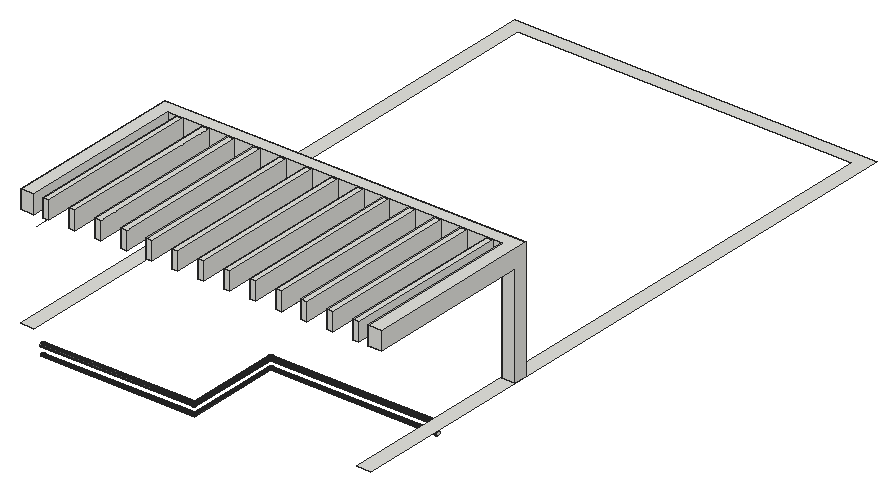
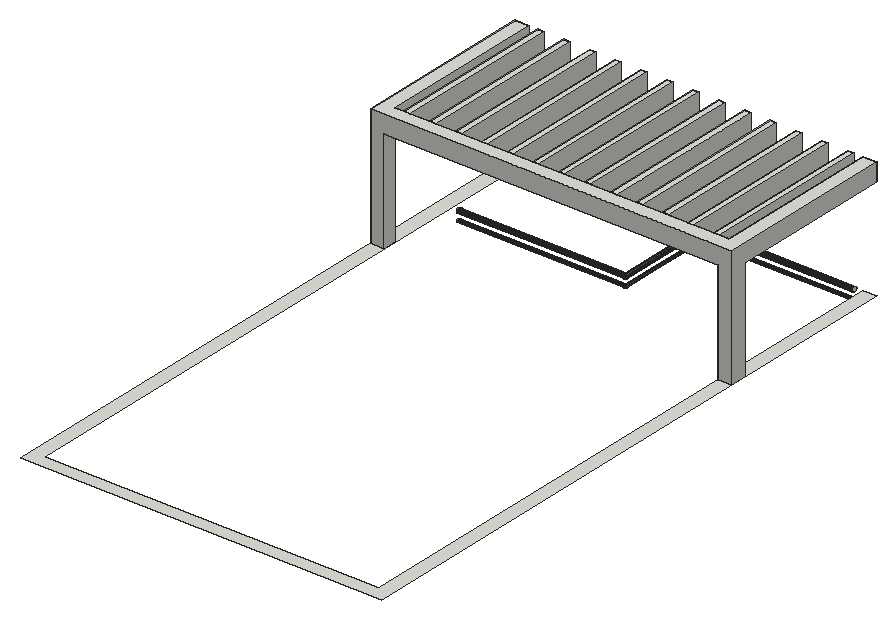
# SketchUp Ruby script. Lengths in inches.
U = 1.inch
M = Sketchup.active_model
def pt(a) = Geom::Point3d.new(a.map { |v| v * U })
def face(e, loops, mat)
  f = e.add_face(loops[0].map { |a| pt(a) })
  loops[1..].each { |l| e.add_face(l.map { |a| pt(a) }).erase! }
  f.material = f.back_material = mat if mat
  f
end
# faces: each face lists its corners as indices into pts; further lists are holes
def faces(e, pts, list, mat = nil) = list.each { |f| face(e, (f[0].is_a?(Array) ? f : [f]).map { |l| l.map { |i| pts[i] } }, mat) }
# xy, xz, yz: faces in a plane at the given z, y or x. An outline is a flat list of corners, or four numbers for a rectangle; further outlines are holes
def ring(l) = l.size == 4 ? [[l[0], l[1]], [l[2], l[1]], [l[2], l[3]], [l[0], l[3]]] : l.each_slice(2).to_a
def flat(e, list, mat, &to3) = list.each { |f| face(e, (f[0].is_a?(Array) ? f : [f]).map { |l| ring(l).map { |u, v| to3.(u, v) } }, mat) }
def xy(e, z, list, mat = nil) = flat(e, list, mat) { |x, y| [x, y, z] }
def xz(e, y, list, mat = nil) = flat(e, list, mat) { |x, z| [x, y, z] }
def yz(e, x, list, mat = nil) = flat(e, list, mat) { |y, z| [x, y, z] }
def lines(e, pts, list) = list.each { |a, b| e.add_line(pt(pts[a]), pt(pts[b])) }
# prism: a flat outline (further loops are holes) pulled along v
def prism(e, loops, v, mat = nil)
  f = face(e, loops, mat); d = Geom::Vector3d.new(v.map { |x| x * U })
  f.pushpull(f.normal.samedirection?(d) ? d.length : -d.length)
end
def box(e, o, s, mat = nil) = prism(e, [[o, [o[0] + s[0], o[1], o[2]], [o[0] + s[0], o[1] + s[1], o[2]], [o[0], o[1] + s[1], o[2]]]], [0, 0, s[2]], mat)
def at(x, y, z, deg = 0) = Geom::Transformation.translation(pt([x, y, z])) * Geom::Transformation.rotation(ORIGIN, Z_AXIS, deg.degrees)
def axes(o, x, y, z) = Geom::Transformation.new([*x, 0, *y, 0, *z, 0, *pt(o).to_a, 1])
def part(name) = M.definitions.add(name)
# library, detail: a bought-in or finely detailed component or shape, given as its bounding box
def library(name, o, s) = part(name).tap { |d| box(d.entities, o, s) }
def detail(e, o, s) = box(e.add_group.entities, o, s)
def put(e, d, t, mat = nil) = e.add_instance(d, t).tap { |i| i.material = mat if mat }
def group(e, t, mat = nil) = e.add_group.tap { |g| g.transformation = t; g.material = mat if mat }.entities
root = M.entities
M.materials.add("[Color M05]").color = [114, 114, 114]
xy(root,307.1,[[231,223.5,240,223.5,240,643.5,0,643.5,0,232.5,9,232.5,9,634.5,231,634.5],[0,341.375,9,352.5],[231,343.5,240,352.5]])
xy(root,375.1,[[0,232.5,9,341.375],[231,232.5,240,343.5],[9,343.5,231,352.5]])
xy(root,387.1,[[0,232.5,9,232.5,9,343.5,231,343.5,231,232.5,240,232.5,240,352.5,0,352.5]])
xz(root,232.5,[[0,375.1,9,387.1],[231,375.1,240,387.1]])
xz(root,341.375,[[0,307.1,9,375.1]])
xz(root,343.5,[[231,307.1,240,375.1],[9,375.1,15,387.1],[19,375.1,231,387.1]])
xz(root,352.5,[[0,307.1,0,387.1,240,387.1,240,307.1,231,307.1,231,375.1,9,375.1,9,307.1]])
yz(root,0,[[341.375,307.1,341.375,375.1,232.5,375.1,232.5,387.1,352.5,387.1,352.5,307.1]])
yz(root,9,[[341.375,307.1,352.5,307.1,352.5,375.1,343.5,375.1,343.5,387.1,232.5,387.1,232.5,375.1,341.375,375.1]])
yz(root,18,[[228,295.92,227.74,295.95,227.5,296.05,227.29,296.21,227.13,296.42,227.03,296.66,227,296.92,227.03,297.18,227.13,297.42,227.29,297.625,227.5,297.78,227.74,297.88,228,297.92,228.26,297.88,228.5,297.78,228.71,297.625,228.87,297.42,228.97,297.18,229,296.92,228.97,296.66,228.87,296.42,228.71,296.21,228.5,296.05,228.26,295.95],[228,301.42,227.61,301.47,227.25,301.62,226.9375,301.86,226.7,302.17,226.55,302.53,226.5,302.92,226.55,303.31,226.7,303.67,226.9375,303.98,227.25,304.22,227.61,304.37,228,304.42,228.39,304.37,228.75,304.22,229.0625,303.98,229.3,303.67,229.45,303.31,229.5,302.92,229.45,302.53,229.3,302.17,229.0625,301.86,228.75,301.62,228.39,301.47]])
yz(root,231,[[291,295.92,291.26,295.95,291.5,296.05,291.71,296.21,291.87,296.42,291.97,296.66,292,296.92,291.97,297.18,291.87,297.42,291.71,297.625,291.5,297.78,291.26,297.88,291,297.92,290.74,297.88,290.5,297.78,290.29,297.625,290.13,297.42,290.03,297.18,290,296.92,290.03,296.66,290.13,296.42,290.29,296.21,290.5,296.05,290.74,295.95],[291,301.42,291.39,301.47,291.75,301.62,292.0625,301.86,292.3,302.17,292.45,302.53,292.5,302.92,292.45,303.31,292.3,303.67,292.0625,303.98,291.75,304.22,291.39,304.37,291,304.42,290.61,304.37,290.25,304.22,289.9375,303.98,289.7,303.67,289.55,303.31,289.5,302.92,289.55,302.53,289.7,302.17,289.9375,301.86,290.25,301.62,290.61,301.47],[343.5,307.1,352.5,375.1],[232.5,375.1,343.5,387.1]])
yz(root,240,[[343.5,307.1,352.5,307.1,352.5,387.1,232.5,387.1,232.5,375.1,343.5,375.1]])
p = [[119.5,228,295.92],[119.76,227.74,295.95],[18,227.74,295.95],[18,228,295.92],[119.5,291,295.92],[119.76,290.74,295.95],
  [119.24,228.26,295.95],[18,228.26,295.95],[119.24,291.26,295.95],[231,291,295.92],[231,290.74,295.95],[231,291.26,295.95],
  [120,227.5,296.05],[18,227.5,296.05],[120,290.5,296.05],[119,228.5,296.05],[18,228.5,296.05],[119,291.5,296.05],
  [231,290.5,296.05],[231,291.5,296.05],[120.21,227.29,296.21],[18,227.29,296.21],[120.21,290.29,296.21],[118.79,228.71,296.21],
  [18,228.71,296.21],[118.79,291.71,296.21],[231,290.29,296.21],[231,291.71,296.21],[120.37,227.13,296.42],[18,227.13,296.42],
  [120.37,290.13,296.42],[118.63,228.87,296.42],[18,228.87,296.42],[118.63,291.87,296.42],[231,290.13,296.42],[231,291.87,296.42],
  [120.47,227.03,296.66],[18,227.03,296.66],[120.47,290.03,296.66],[118.53,228.97,296.66],[18,228.97,296.66],[118.53,291.97,296.66],
  [231,290.03,296.66],[231,291.97,296.66],[120.5,227,296.92],[18,227,296.92],[120.5,290,296.92],[118.5,229,296.92],
  [18,229,296.92],[118.5,292,296.92],[231,290,296.92],[231,292,296.92],[120.47,227.03,297.18],[18,227.03,297.18],
  [120.47,290.03,297.18],[118.53,228.97,297.18],[18,228.97,297.18],[118.53,291.97,297.18],[231,290.03,297.18],[231,291.97,297.18],
  [120.37,227.13,297.42],[18,227.13,297.42],[120.37,290.13,297.42],[118.63,228.87,297.42],[18,228.87,297.42],[118.63,291.87,297.42],
  [231,290.13,297.42],[231,291.87,297.42],[120.21,227.29,297.625],[18,227.29,297.625],[120.21,290.29,297.625],[118.79,228.71,297.625],
  [18,228.71,297.625],[118.79,291.71,297.625],[231,290.29,297.625],[231,291.71,297.625],[120,227.5,297.78],[18,227.5,297.78],
  [120,290.5,297.78],[119,228.5,297.78],[18,228.5,297.78],[119,291.5,297.78],[231,290.5,297.78],[231,291.5,297.78],
  [119.76,227.74,297.88],[18,227.74,297.88],[119.76,290.74,297.88],[119.24,228.26,297.88],[18,228.26,297.88],[119.24,291.26,297.88],
  [231,290.74,297.88],[231,291.26,297.88],[119.5,228,297.92],[18,228,297.92],[119.5,291,297.92],[231,291,297.92],
  [119.5,228,301.42],[119.89,227.61,301.47],[18,227.61,301.47],[18,228,301.42],[119.5,291,301.42],[119.89,290.61,301.47],
  [119.11,228.39,301.47],[18,228.39,301.47],[119.11,291.39,301.47],[231,291,301.42],[231,290.61,301.47],[231,291.39,301.47],
  [120.25,227.25,301.62],[18,227.25,301.62],[120.25,290.25,301.62],[118.75,228.75,301.62],[18,228.75,301.62],[118.75,291.75,301.62],
  [231,290.25,301.62],[231,291.75,301.62],[120.5625,226.9375,301.86],[18,226.9375,301.86],[120.5625,289.9375,301.86],[118.4375,229.0625,301.86],
  [18,229.0625,301.86],[118.4375,292.0625,301.86],[231,289.9375,301.86],[231,292.0625,301.86],[120.8,226.7,302.17],[18,226.7,302.17],
  [120.8,289.7,302.17],[118.2,229.3,302.17],[18,229.3,302.17],[118.2,292.3,302.17],[231,289.7,302.17],[231,292.3,302.17],
  [120.95,226.55,302.53],[18,226.55,302.53],[120.95,289.55,302.53],[118.05,229.45,302.53],[18,229.45,302.53],[118.05,292.45,302.53],
  [231,289.55,302.53],[231,292.45,302.53],[121,226.5,302.92],[18,226.5,302.92],[121,289.5,302.92],[118,229.5,302.92],
  [18,229.5,302.92],[118,292.5,302.92],[231,289.5,302.92],[231,292.5,302.92],[120.95,226.55,303.31],[18,226.55,303.31],
  [120.95,289.55,303.31],[118.05,229.45,303.31],[18,229.45,303.31],[118.05,292.45,303.31],[231,289.55,303.31],[231,292.45,303.31],
  [120.8,226.7,303.67],[18,226.7,303.67],[120.8,289.7,303.67],[118.2,229.3,303.67],[18,229.3,303.67],[118.2,292.3,303.67],
  [231,289.7,303.67],[231,292.3,303.67],[120.5625,226.9375,303.98],[18,226.9375,303.98],[120.5625,289.9375,303.98],[118.4375,229.0625,303.98],
  [18,229.0625,303.98],[118.4375,292.0625,303.98],[231,289.9375,303.98],[231,292.0625,303.98],[120.25,227.25,304.22],[18,227.25,304.22],
  [120.25,290.25,304.22],[118.75,228.75,304.22],[18,228.75,304.22],[118.75,291.75,304.22],[231,290.25,304.22],[231,291.75,304.22],
  [119.89,227.61,304.37],[18,227.61,304.37],[119.89,290.61,304.37],[119.11,228.39,304.37],[18,228.39,304.37],[119.11,291.39,304.37],
  [231,290.61,304.37],[231,291.39,304.37],[119.5,228,304.42],[18,228,304.42],[119.5,291,304.42],[231,291,304.42],
  [18,232.5,375.1],[18,223.5,375.1]]
faces(root,p,[[0,1,2,3],[4,5,1,0],[6,0,3,7],[8,4,0,6],[9,10,5,4],[11,9,4,8],[1,12,13,2],[5,14,12,1],
  [15,6,7,16],[17,8,6,15],[10,18,14,5],[19,11,8,17],[12,20,21,13],[14,22,20,12],[23,15,16,24],[25,17,15,23],
  [18,26,22,14],[27,19,17,25],[20,28,29,21],[22,30,28,20],[31,23,24,32],[33,25,23,31],[26,34,30,22],[35,27,25,33],
  [28,36,37,29],[30,38,36,28],[39,31,32,40],[41,33,31,39],[34,42,38,30],[43,35,33,41],[36,44,45,37],[38,46,44,36],
  [47,39,40,48],[49,41,39,47],[42,50,46,38],[51,43,41,49],[44,52,53,45],[46,54,52,44],[55,47,48,56],[57,49,47,55],
  [50,58,54,46],[59,51,49,57],[52,60,61,53],[54,62,60,52],[63,55,56,64],[65,57,55,63],[58,66,62,54],[67,59,57,65],
  [60,68,69,61],[62,70,68,60],[71,63,64,72],[73,65,63,71],[66,74,70,62],[75,67,65,73],[68,76,77,69],[70,78,76,68],
  [79,71,72,80],[81,73,71,79],[74,82,78,70],[83,75,73,81],[76,84,85,77],[78,86,84,76],[87,79,80,88],[89,81,79,87],
  [82,90,86,78],[91,83,81,89],[84,92,93,85],[86,94,92,84],[92,87,88,93],[94,89,87,92],[90,95,94,86],[95,91,89,94],
  [96,97,98,99],[100,101,97,96],[102,96,99,103],[104,100,96,102],[105,106,101,100],[107,105,100,104],[97,108,109,98],[101,110,108,97],
  [111,102,103,112],[113,104,102,111],[106,114,110,101],[115,107,104,113],[108,116,117,109],[110,118,116,108],[119,111,112,120],[121,113,111,119],
  [114,122,118,110],[123,115,113,121],[116,124,125,117],[118,126,124,116],[127,119,120,128],[129,121,119,127],[122,130,126,118],[131,123,121,129],
  [124,132,133,125],[126,134,132,124],[135,127,128,136],[137,129,127,135],[130,138,134,126],[139,131,129,137],[132,140,141,133],[134,142,140,132],
  [143,135,136,144],[145,137,135,143],[138,146,142,134],[147,139,137,145],[140,148,149,141],[142,150,148,140],[151,143,144,152],[153,145,143,151],
  [146,154,150,142],[155,147,145,153],[148,156,157,149],[150,158,156,148],[159,151,152,160],[161,153,151,159],[154,162,158,150],[163,155,153,161],
  [156,164,165,157],[158,166,164,156],[167,159,160,168],[169,161,159,167],[162,170,166,158],[171,163,161,169],[164,172,173,165],[166,174,172,164],
  [175,167,168,176],[177,169,167,175],[170,178,174,166],[179,171,169,177],[172,180,181,173],[174,182,180,172],[183,175,176,184],[185,177,175,183],
  [178,186,182,174],[187,179,177,185],[180,188,189,181],[182,190,188,180],[188,183,184,189],[190,185,183,188],[186,191,190,182],[191,187,185,190]],"[Color M05]")
lines(root,p,[[192,193]])
g1 = group(root,at(15,343.5,375.1))
box(g1,[0,-111,0],[4,111,12])
g2 = group(root,at(49.33,343.5,375.1))
box(g2,[0,-111,0],[4,111,12])
g3 = group(root,at(32.17,343.5,375.1))
box(g3,[0,-111,0],[4,111,12])
g4 = group(root,at(66.5,343.5,375.1))
box(g4,[0,-111,0],[4,111,12])
g5 = group(root,at(83.67,343.5,375.1))
box(g5,[0,-111,0],[4,111,12])
g6 = group(root,at(100.83,343.5,375.1))
box(g6,[0,-111,0],[4,111,12])
g7 = group(root,at(118,343.5,375.1))
box(g7,[0,-111,0],[4,111,12])
g8 = group(root,at(135.17,343.5,375.1))
box(g8,[0,-111,0],[4,111,12])
g9 = group(root,at(152.33,343.5,375.1))
box(g9,[0,-111,0],[4,111,12])
g10 = group(root,at(169.5,343.5,375.1))
box(g10,[0,-111,0],[4,111,12])
g11 = group(root,at(186.67,343.5,375.1))
box(g11,[0,-111,0],[4,111,12])
g12 = group(root,at(203.83,343.5,375.1))
box(g12,[0,-111,0],[4,111,12])
g13 = group(root,at(221,343.5,375.1))
box(g13,[0,-111,0],[4,111,12])
